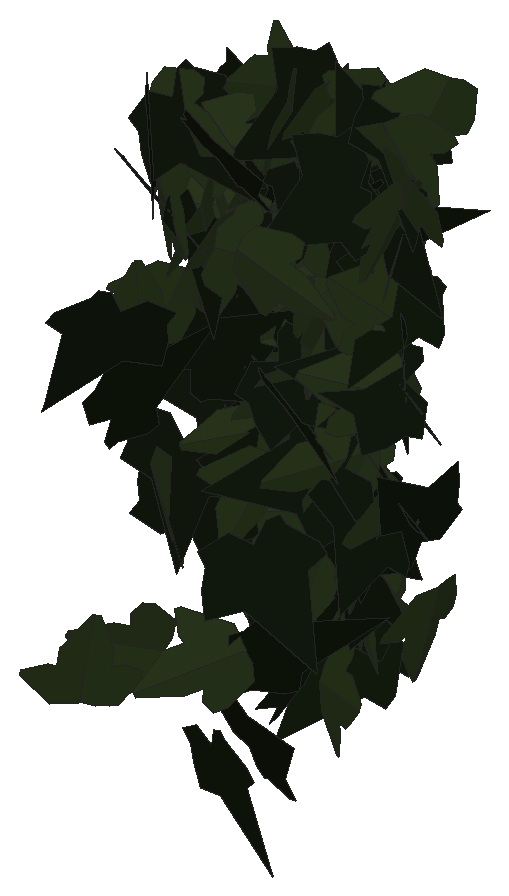
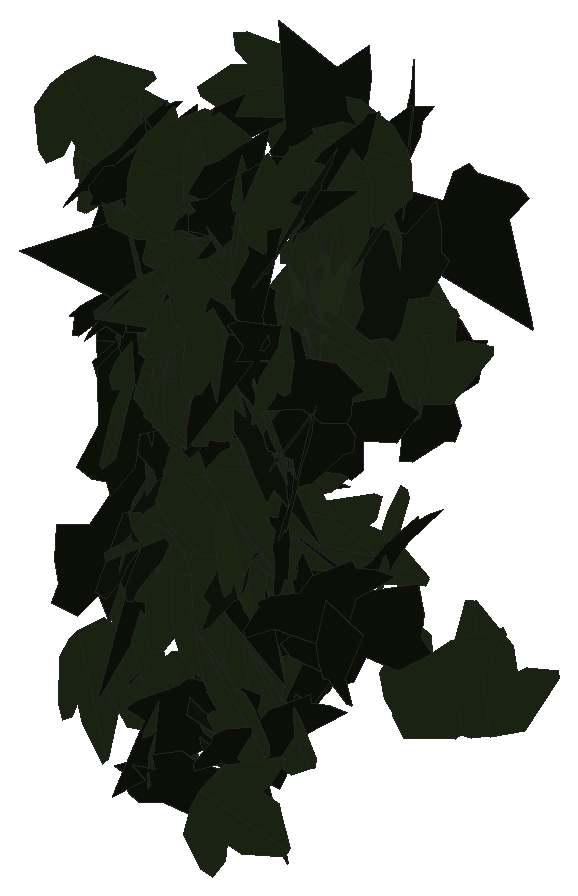
# SketchUp Ruby script. Lengths in inches.
U = 1.inch
M = Sketchup.active_model
def pt(a) = Geom::Point3d.new(a.map { |v| v * U })
def face(e, loops, mat)
  f = e.add_face(loops[0].map { |a| pt(a) })
  loops[1..].each { |l| e.add_face(l.map { |a| pt(a) }).erase! }
  f.material = f.back_material = mat if mat
  f
end
# faces: each face lists its corners as indices into pts; further lists are holes
def faces(e, pts, list, mat = nil) = list.each { |f| face(e, (f[0].is_a?(Array) ? f : [f]).map { |l| l.map { |i| pts[i] } }, mat) }
# xy, xz, yz: faces in a plane at the given z, y or x. An outline is a flat list of corners, or four numbers for a rectangle; further outlines are holes
def ring(l) = l.size == 4 ? [[l[0], l[1]], [l[2], l[1]], [l[2], l[3]], [l[0], l[3]]] : l.each_slice(2).to_a
def flat(e, list, mat, &to3) = list.each { |f| face(e, (f[0].is_a?(Array) ? f : [f]).map { |l| ring(l).map { |u, v| to3.(u, v) } }, mat) }
def xy(e, z, list, mat = nil) = flat(e, list, mat) { |x, y| [x, y, z] }
def xz(e, y, list, mat = nil) = flat(e, list, mat) { |x, z| [x, y, z] }
def yz(e, x, list, mat = nil) = flat(e, list, mat) { |y, z| [x, y, z] }
def lines(e, pts, list) = list.each { |a, b| e.add_line(pt(pts[a]), pt(pts[b])) }
# prism: a flat outline (further loops are holes) pulled along v
def prism(e, loops, v, mat = nil)
  f = face(e, loops, mat); d = Geom::Vector3d.new(v.map { |x| x * U })
  f.pushpull(f.normal.samedirection?(d) ? d.length : -d.length)
end
def box(e, o, s, mat = nil) = prism(e, [[o, [o[0] + s[0], o[1], o[2]], [o[0] + s[0], o[1] + s[1], o[2]], [o[0], o[1] + s[1], o[2]]]], [0, 0, s[2]], mat)
def at(x, y, z, deg = 0) = Geom::Transformation.translation(pt([x, y, z])) * Geom::Transformation.rotation(ORIGIN, Z_AXIS, deg.degrees)
def axes(o, x, y, z) = Geom::Transformation.new([*x, 0, *y, 0, *z, 0, *pt(o).to_a, 1])
def part(name) = M.definitions.add(name)
# library, detail: a bought-in or finely detailed component or shape, given as its bounding box
def library(name, o, s) = part(name).tap { |d| box(d.entities, o, s) }
def detail(e, o, s) = box(e.add_group.entities, o, s)
def put(e, d, t, mat = nil) = e.add_instance(d, t).tap { |i| i.material = mat if mat }
def group(e, t, mat = nil) = e.add_group.tap { |g| g.transformation = t; g.material = mat if mat }.entities
root = M.entities
M.materials.add("efeu1").color = [18, 25, 13]
M.materials.add("efeu2").color = [43, 57, 29]
c1 = part("ivyleaf_9")
p = [[1.54,2.16,1.25],[1.36,2.04,1.19],[-0.21,0.99,0.68],[-0.71,1.11,0.82],[-0.85,0.86,0.67],[-0.8,0.17,0.21],
  [-0.9,-0.01,0.1],[-0.67,-0.16,-0.02],[-0.08,-0.08,-0.05],[-0.03,-0.6,-0.4],[0.65,-0.88,-0.66],[0.83,-0.6,-0.49],
  [1.29,-0.42,-0.43],[1.8125,-0.07,-0.26],[1.21,0.44,0.15]]
faces(c1.entities,p,[[0,1,2,3,4,5,6,7,8,9,10,11,12,13,14]],"efeu1")
c2 = part("ivyleaf_10")
p = [[0,0.5,-0.03],[-0.0625,2.02,-0.43],[-0.19,2.01,-0.46],[-0.54,1.05,-0.29],[-0.52,0.625,-0.18],[-0.83,0.76,-0.28],
  [-1.16,0.64,-0.33],[-1.15,0.33,-0.24],[-0.77,-0.39,0.02],[-0.3,-0.51,0.16],[0.04,-0.48,0.23],[-0.02,2.01,-0.4375],
  [-0.06,2.01,-0.43],[0.04,-0.49,0.23],[0.67,-0.49,0.14],[1.38,0.36,-0.2],[1.375,0.51,-0.24],[0.81,0.65,-0.19],
  [0.62,0.59,-0.15],[0.6,1.09,-0.28],[0.5,1.23,-0.31]]
faces(c2.entities,p,[[0,1,2,3,4,5,6,7,8,9,10],[11,12,0,13,14,15,16,17,18,19,20]],"efeu2")
put(root,c1,axes([18.06,224.125,208.98],[-0.01391,0.03121,0.49883],[-0.2386,0.43807,-0.03406],[-0.43918,-0.23899,0.00271]))
put(root,c1,axes([17.82,224.65,209.74],[-0.1901,-0.4622,-0.01517],[0.00198,0.01558,-0.49975],[0.46245,-0.19007,-0.00409]))
put(root,c2,axes([17.95,222.78,211.19],[-0.31818,-0.37826,-0.07536],[-0.04879,-0.05744,0.49429],[-0.3826,0.3219,-0.00036]))
put(root,c2,axes([17.9,221.86,207.3],[-0.37151,-0.33269,0.03604],[0.02825,0.02248,0.49869],[-0.33344,0.37257,0.0021]))
put(root,c1,axes([17.58,223.4375,212.44],[0.12943,-0.28938,0.38666],[0.26736,-0.29043,-0.30686],[0.4022,0.28619,0.07956]))
put(root,c2,axes([17.55,224.12,212.06],[0.11112,-0.14043,-0.46683],[0.47707,-0.06718,0.13376],[-0.1003,-0.47515,0.11906]))
put(root,c2,axes([18.23,222.51,207.6],[-0.11023,-0.14853,-0.46453],[-0.2849,-0.36692,0.18493],[-0.39583,0.30546,-0.00374]))
put(root,c2,axes([18.21,223.04,211.77],[-0.26597,-0.38738,0.17088],[-0.08938,-0.14587,-0.46982],[0.41385,-0.28046,0.00835]))
put(root,c2,axes([18.04,224.69,212.23],[-0.00323,0.33062,-0.37508],[-0.01008,-0.37505,-0.33051],[-0.49989,0.00542,0.00909]))
put(root,c1,axes([17.93,223.48,209.53],[0.01314,-0.49109,0.09307],[0.01459,-0.09268,-0.49112],[0.49961,0.01562,0.0119]))
put(root,c1,axes([17.84,224.65,211.09],[0.13457,-0.07798,-0.4752],[0.43428,-0.19355,0.15474],[-0.20808,-0.45438,0.01564]))
put(root,c1,axes([17.99,223.54,208.6],[-0.22356,-0.06502,0.44248],[0.44577,-0.07247,0.21457],[0.03623,0.49043,0.09037]))
put(root,c1,axes([17.92,222.95,213.77],[0.05224,-0.08497,-0.48995],[0.46894,-0.15548,0.07696],[-0.16543,-0.46755,0.06345]))
put(root,c1,axes([17.8125,224.19,211.47],[0.40854,-0.13619,0.25406],[0.24568,-0.06599,-0.43045],[0.15077,0.47655,0.013]))
put(root,c2,axes([18.26,222.72,209.51],[-0.28195,0.40988,0.05002],[-0.02911,0.04069,-0.49749],[-0.41189,-0.28345,0.00092]))
put(root,c1,axes([17.95,224.48,212.09],[-0.05685,-0.19259,-0.4579],[0.34535,0.31598,-0.17577],[0.35708,-0.33626,0.0971]))
put(root,c1,axes([18.1,223.16,213.88],[0.15552,-0.30654,-0.3631],[-0.08133,0.35925,-0.33812],[0.46819,0.16423,0.06188]))
put(root,c2,axes([17.91,223.29,213.7],[-0.09678,0.01653,-0.49027],[0.45247,-0.19003,-0.09573],[-0.18949,-0.46219,0.02182]))
put(root,c1,axes([18.15,222.09,210.59],[0.04154,0.03134,0.49728],[0.33791,0.36495,-0.05123],[-0.36618,0.34033,0.00914]))
put(root,c1,axes([18.07,224.13,211.43],[0.29374,-0.39325,-0.09524],[-0.04492,0.08526,-0.49062],[0.40212,0.29679,0.01476]))
put(root,c2,axes([18.4,223.18,212.625],[0.0467,-0.41452,-0.27567],[-0.02682,0.27438,-0.41713],[0.49709,0.05374,0.0034]))
put(root,c2,axes([18.09,223.98,212.17],[-0.17648,-0.00632,0.46778],[0.38989,-0.27828,0.14333],[0.25854,0.41535,0.10315]))
put(root,c2,axes([18.08,223.06,212.8],[-0.11914,0.05053,-0.48296],[0.29143,-0.39033,-0.11273],[-0.38843,-0.30836,0.06355]))
put(root,c1,axes([18.47,224.61,211.29],[-0.37999,0.23331,-0.22622],[0.19248,-0.11886,-0.4459],[-0.26184,-0.42596,0.00052]))
put(root,c1,axes([18.14,224.44,213.35],[0.09216,-0.40164,0.28318],[0.04923,-0.27912,-0.4119],[0.48896,0.10381,-0.0119]))
put(root,c2,axes([18.4,223.83,212.2],[0.06041,-0.49434,0.04446],[0.0108,-0.04347,-0.49799],[0.49622,0.06113,0.00543]))
put(root,c1,axes([18.07,224.58,210.4375],[0.04402,-0.02574,-0.49739],[0.48753,-0.09992,0.04831],[-0.10189,-0.48924,0.0163]))
put(root,c2,axes([18.36,224.5625,213.52],[-0.05767,0.24345,0.4329],[0.11981,-0.41612,0.24997],[0.482,0.13256,-0.01034]))
put(root,c2,axes([18.39,224.48,211.45],[0.34023,-0.36262,0.05241],[0.03285,-0.04103,-0.49723],[0.36491,0.34179,-0.00409]))
put(root,c2,axes([18.53,224.34,211.49],[-0.37197,-0.32722,0.06757],[-0.04635,-0.04961,-0.49537],[0.33089,-0.37479,0.00658]))
put(root,c1,axes([18.62,221.54,212.18],[0.03438,0.26818,-0.42059],[-0.06367,-0.41578,-0.27032],[-0.49474,0.07215,0.00556]))
put(root,c2,axes([18.75,224.04,209.79],[-0.0862,-0.04576,0.49038],[-0.31876,-0.37432,-0.09096],[0.37545,-0.32831,0.03535]))
put(root,c2,axes([18.42,223.91,212.52],[0.22308,-0.36624,0.25711],[0.14635,-0.21177,-0.42864],[0.42287,0.2665,0.01271]))
put(root,c1,axes([18.3,223.34,212.4],[0.13837,-0.43133,0.21168],[0.0469,-0.20711,-0.45267],[0.47818,0.14513,-0.01686]))
put(root,c1,axes([18.46,224.53,208.05],[-0.15806,-0.47234,-0.04373],[0.0209,0.03912,-0.49803],[0.4739,-0.15926,0.00738]))
put(root,c1,axes([18.25,223.3,210.67],[-0.03073,-0.00895,0.49897],[0.49741,-0.04107,0.0299],[0.04045,0.49823,0.01143]))
put(root,c2,axes([18.65,224.83,207.3],[-0.12624,-0.30457,0.3759],[-0.01443,-0.38594,-0.31756],[0.48359,-0.09102,0.08865]))
put(root,c2,axes([18.3,223.48,213.35],[-0.08444,-0.07794,-0.48661],[0.43558,0.21914,-0.11069],[0.23053,-0.44261,0.03089]))
put(root,c2,axes([18.66,223.28,212.5],[0.12797,-0.48014,0.05555],[0.0076,-0.05546,-0.49686],[0.48329,0.12801,-0.0069]))
put(root,c2,axes([18.375,224.1,207.72],[0.37705,-0.15621,-0.28884],[0.26388,-0.11762,0.40808],[-0.19544,-0.46018,-0.00626]))
put(root,c2,axes([18.71,224.52,210.04],[0.10057,-0.48748,0.04741],[0.01077,-0.04618,-0.49775],[0.48966,0.10114,0.00121]))
put(root,c1,axes([18.94,224.45,213.06],[-0.18368,-0.12444,0.44808],[-0.38532,-0.22901,-0.22155],[0.26037,-0.4267,-0.01176]))
put(root,c1,axes([18.93,224.34,212.3],[0.14648,-0.14558,0.45536],[-0.24874,0.3835,0.20263],[-0.40825,-0.2859,0.03992]))
put(root,c2,axes([18.83,224.55,212.08],[-0.1472,-0.46998,0.08632],[-0.02027,-0.0841,-0.49246],[0.47741,-0.14848,0.0057]))
put(root,c2,axes([18.8,224.17,213.59],[0.08389,-0.38615,-0.30635],[-0.00954,0.30943,-0.39264],[0.49282,0.07172,0.04455]))
put(root,c2,axes([18.89,224.47,210.35],[0.44435,0.03637,-0.22634],[-0.22478,-0.02779,-0.44576],[-0.045,0.4979,-0.00834]))
put(root,c2,axes([18.52,224.59,208],[0.35812,-0.15987,-0.31015],[0.28195,-0.12922,0.39218],[-0.20555,-0.45579,-0.00241]))
put(root,c1,axes([18.65,224.49,212.13],[-0.28484,-0.17925,-0.36977],[0.31996,0.18558,-0.33643],[0.25786,-0.42829,0.00898]))
put(root,c1,axes([18.97,224.63,213.51],[-0.18501,-0.27509,0.3743],[-0.20926,-0.31034,-0.33151],[0.41471,-0.27931,-0.0003]))
put(root,c1,axes([18.86,224.32,212.35],[0.43281,0.14078,-0.20702],[-0.19613,-0.06631,-0.45512],[-0.1556,0.47517,-0.00218]))
put(root,c2,axes([19.02,224.51,212.73],[-0.24145,-0.33894,0.27717],[-0.06828,-0.28351,-0.40616],[0.43248,-0.23398,0.09062]))
put(root,c2,axes([18.82,223.14,212.35],[0.00931,-0.2776,-0.41575],[0.19873,0.38361,-0.25169],[0.45871,-0.16056,0.11748]))
put(root,c2,axes([19.12,224.55,210.09],[-0.23467,-0.22531,-0.37969],[-0.24908,-0.28747,0.32453],[-0.36454,0.34146,0.02268]))
put(root,c2,axes([19.02,224.82,211.61],[-0.02814,-0.15999,0.47288],[0.02645,-0.47344,-0.15861],[0.49851,0.01609,0.03511]))
put(root,c1,axes([18.72,224.34,209.63],[0.27871,-0.38288,0.1604],[0.09505,-0.1292,-0.47357],[0.40409,0.29447,0.00076]))
put(root,c1,axes([19.32,223.99,209.48],[0.13681,0.0602,-0.47714],[-0.44033,-0.18378,-0.14944],[-0.19337,0.46109,0.00273]))
put(root,c2,axes([18.82,223.87,208.45],[-0.04573,-0.01926,-0.49753],[0.32055,-0.38345,-0.01462],[-0.38099,-0.32031,0.04742]))
put(root,c2,axes([19.23,223.25,209.76],[-0.22513,-0.38611,0.22413],[-0.06689,-0.21901,-0.44448],[0.44141,-0.23012,0.04696]))
put(root,c2,axes([19.17,224.38,213.8],[0.05287,-0.4972,0.00042],[-0.00039,-0.00046,-0.5],[0.4972,0.05287,-0.00044]))
put(root,c2,axes([19.48,224.52,211.39],[0.11406,0.09201,-0.47804],[-0.47672,-0.07834,-0.12883],[-0.0986,0.48518,0.06985]))
put(root,c1,axes([18.85,223,213.49],[0.00147,-0.2279,0.44504],[0.31332,-0.3464,-0.17842],[0.38965,0.27941,0.14179]))
put(root,c2,axes([19,224.33,212.47],[-0.29899,-0.20363,-0.34517],[0.30185,0.16885,-0.36108],[0.26362,-0.42429,0.02196]))
put(root,c2,axes([19.25,223.91,209.9],[0.16636,-0.46218,-0.09333],[-0.0312,0.08796,-0.49121],[0.47048,0.16926,0.00042]))
put(root,c2,axes([19.22,224.29,211.43],[-0.13452,-0.29638,0.37956],[0.1126,-0.40252,-0.2744],[0.46821,0.01165,0.17504]))
put(root,c1,axes([19.53,223.65,207.39],[-0.28898,0.40736,0.02331],[-0.01352,0.01899,-0.49946],[-0.40781,-0.2893,0.00004]))
put(root,c2,axes([19.18,224.56,211.28],[-0.096,0.38894,-0.29918],[0.05583,-0.29421,-0.4004],[-0.48751,-0.11028,0.01306]))
put(root,c2,axes([19.37,224.46,209.17],[-0.12926,-0.46906,0.11522],[-0.03419,-0.11009,-0.48653],[0.48179,-0.13365,-0.00362]))
put(root,c2,axes([19.5,224.41,211.27],[0.06599,0.07364,-0.49013],[-0.35404,-0.33902,-0.0986],[-0.34685,0.36006,0.0074]))
put(root,c1,axes([19.46,223.68,207.57],[-0.34191,0.28777,-0.22424],[-0.16989,0.14638,0.44689],[0.32285,0.38179,-0.00232]))
put(root,c2,axes([19.25,223.85,207.76],[-0.3407,-0.35144,0.10205],[0.06938,0.07487,0.48947],[-0.35932,0.34768,-0.00224]))
put(root,c1,axes([19.12,224.41,208.04],[0.03068,-0.2969,-0.40114],[0.09241,0.39832,-0.28775],[0.49043,-0.05648,0.07931]))
put(root,c2,axes([19.46,224.74,213.67],[-0.04066,-0.24872,0.43184],[-0.06656,-0.42668,-0.25201],[0.49388,-0.07798,0.00158]))
put(root,c1,axes([19.52,224.61,207.25],[-0.45889,-0.19611,0.03101],[-0.02762,-0.01428,-0.49903],[0.19661,-0.45971,0.00228]))
put(root,c2,axes([19.49,223.35,210.92],[-0.14609,-0.4746,-0.05844],[0.01894,0.05532,-0.49657],[0.47781,-0.1473,0.00182]))
put(root,c2,axes([19.11,223.63,209.11],[0.09403,-0.00935,-0.49099],[0.49026,-0.02713,0.0944],[-0.02841,-0.49918,0.00406]))
put(root,c2,axes([19.46,223.99,209.81],[0.05752,0.42974,0.24903],[0.00623,0.25005,-0.43294],[-0.49664,0.0529,0.02341]))
put(root,c2,axes([19.83,221.8,208.36],[-0.17647,-0.08274,0.46045],[-0.2877,-0.36886,-0.17655],[0.3689,-0.32725,0.08258]))
put(root,c2,axes([19.27,224.31,211.47],[0.35642,-0.03769,0.34863],[0.34816,-0.0212,-0.35824],[0.04179,0.49813,0.01113]))
put(root,c2,axes([19.5,223.92,211.44],[0.20464,-0.39763,0.22363],[0.12989,-0.18417,-0.44633],[0.43732,0.24077,0.02792]))
put(root,c2,axes([19.52,223.76,211.7],[-0.02955,0.44421,-0.2276],[0.01879,-0.22685,-0.44518],[-0.49877,-0.03487,-0.00329]))
put(root,c2,axes([19.61,224.33,207.99],[-0.21593,0.44443,0.07651],[-0.04346,0.06393,-0.49399],[-0.44887,-0.21998,0.01102]))
put(root,c1,axes([19.58,223.93,212.8],[-0.34404,0.30144,0.20193],[0.15339,-0.13134,0.45741],[0.3288,0.37668,-0.0021]))
put(root,c2,axes([19.5,224.23,212.9],[0.36567,0.32207,0.11207],[0.07977,0.07898,-0.48724],[-0.33155,0.37421,0.00638]))
put(root,c1,axes([19.46,223.27,211.13],[0.17521,-0.2168,-0.41509],[-0.02659,0.43787,-0.23992],[0.46754,0.10614,0.14191]))
put(root,c2,axes([19.44,224.14,212.28],[-0.08703,-0.09898,-0.48232],[0.35538,0.32637,-0.1311],[0.34078,-0.36563,0.01354]))
put(root,c1,axes([19.96,223.59,209.9],[-0.08083,-0.1992,-0.45143],[-0.19853,-0.40565,0.21455],[-0.45172,0.21393,-0.01351]))
put(root,c1,axes([19.46,224.44,210.7],[-0.08295,-0.16367,0.46512],[0.21337,-0.43712,-0.11576],[0.44451,0.17928,0.14236]))
put(root,c2,axes([19.83,223.92,211.48],[-0.13951,0.45102,-0.16467],[-0.05894,0.15409,0.472],[0.47651,0.15111,0.01017]))
put(root,c2,axes([19.68,223.89,209.16],[-0.3346,-0.32874,0.17314],[0.12556,0.11925,0.46906],[-0.34969,0.35737,0.00275]))
put(root,c2,axes([19.46,224.57,209.36],[-0.15448,0.06763,-0.4707],[0.42094,-0.21081,-0.16844],[-0.22124,-0.44831,0.0082]))
put(root,c2,axes([19.55,223.99,206.96],[0.04014,-0.12573,-0.48227],[0.32658,-0.35884,0.12074],[-0.37647,-0.32469,0.05331]))
put(root,c1,axes([19.52,223.27,210.7],[0.1759,-0.33052,0.33138],[0.21469,-0.25759,-0.37088],[0.41589,0.27277,0.0513]))
put(root,c2,axes([19.93,223.625,210],[0.00336,0.04745,0.49773],[-0.01291,-0.49757,0.04753],[0.49982,-0.01318,-0.00212]))
put(root,c1,axes([20.09,224.25,213.02],[-0.36083,-0.32881,0.10807],[0.08658,0.06541,0.48808],[-0.33511,0.37095,0.00974]))
put(root,c2,axes([19.74,224.51,207.92],[-0.4226,-0.01688,0.26668],[0.26721,-0.02945,0.42158],[0.00147,0.49885,0.03391]))
put(root,c1,axes([19.65,221.88,207.14],[0.30718,-0.39407,0.01871],[0.01178,-0.01455,-0.49965],[0.39433,0.30741,0.00035]))
put(root,c1,axes([20.03,223.77,213.24],[-0.23591,-0.27691,0.34303],[-0.168,-0.30323,-0.36032],[0.40759,-0.28526,0.05003]))
put(root,c1,axes([19.95,224.58,209.21],[0.31798,-0.37904,0.07222],[-0.03007,0.06896,0.49431],[-0.38468,-0.31871,0.02107]))
put(root,c1,axes([19.79,224.3,208.34],[-0.03146,-0.37819,0.32555],[0.08068,-0.32576,-0.37064],[0.49244,0.02921,0.08152]))
put(root,c1,axes([20,224.05,209.15],[0.15054,-0.15674,-0.4503],[-0.31639,0.32043,-0.2173],[0.3567,0.35037,-0.0027]))
put(root,c1,axes([19.68,224.17,212.36],[0.21016,0.06627,0.44882],[0.42271,0.15103,-0.22023],[-0.16476,0.47201,0.00745]))
put(root,c1,axes([19.85,224.43,212.21],[0.06748,-0.49482,-0.02448],[0.00047,0.02477,-0.49939],[0.49543,0.06737,0.00381]))
put(root,c1,axes([19.79,222.33,207.05],[-0.02002,-0.12847,0.4828],[0.30063,-0.38901,-0.09104],[0.39902,0.28664,0.09282]))
put(root,c2,axes([20.12,224.29,208.96],[0.03509,0.11146,-0.48615],[-0.08959,-0.47802,-0.11606],[-0.49066,0.09525,-0.01357]))
put(root,c2,axes([20.23,224.21,212.54],[0.27749,-0.37907,-0.17118],[-0.0889,0.14697,-0.46957],[0.40632,0.29104,0.01416]))
put(root,c1,axes([19.97,224.65,213.68],[0.06912,-0.49407,0.03339],[0.00576,-0.03291,-0.49888],[0.49517,0.06935,0.00114]))
put(root,c1,axes([19.91,224.125,212.88],[-0.11842,-0.12845,-0.46848],[0.34721,0.31486,-0.17409],[0.33974,-0.36655,0.01462]))
put(root,c2,axes([20.21,223.95,210.96],[-0.05292,-0.32136,-0.37937],[0.04797,0.37644,-0.32557],[0.49487,-0.07086,-0.00901]))
put(root,c1,axes([20.0625,222.0625,209.625],[-0.01063,-0.3671,-0.3393],[0.06249,0.33574,-0.3652],[0.49597,-0.05017,0.03874]))
put(root,c1,axes([19.99,222.2,208.2],[0.16951,0.10164,0.45928],[0.39562,0.23329,-0.19764],[-0.25447,0.4304,-0.00133]))
put(root,c2,axes([20.22,224.1875,213.74],[-0.41659,-0.21555,-0.17319],[0.15027,0.0864,-0.46899],[0.23211,-0.4428,-0.00721]))
put(root,c1,axes([19.92,224.46,210.64],[0.37878,-0.05886,-0.32103],[0.31423,-0.06717,0.38308],[-0.08822,-0.49196,-0.0139]))
put(root,c2,axes([20.3,223.86,211.79],[-0.08169,0.35714,0.34026],[0.05437,-0.33628,0.36601],[0.49028,0.09679,0.0161]))
put(root,c1,axes([20.04,224.3,211.38],[-0.11719,-0.01761,-0.48575],[0.48569,-0.02396,-0.11631],[-0.01919,-0.49911,0.02272]))
put(root,c1,axes([20.29,224.37,211.96],[-0.15712,-0.43097,0.19894],[-0.06986,-0.18627,-0.45872],[0.4695,-0.17194,-0.00168]))
put(root,c2,axes([20.3,223.84,209.29],[0.12315,-0.42875,0.22584],[0.0921,-0.20807,-0.44523],[0.47576,0.15126,0.02773]))
put(root,c2,axes([20.43,224.69,214.09],[-0.22568,-0.37882,0.23572],[-0.04174,-0.24507,-0.43382],[0.44421,-0.21549,0.07899]))
put(root,c1,axes([20.19,223.83,209.36],[-0.05949,-0.43349,0.24197],[0.0285,-0.24628,-0.43421],[0.49563,-0.03787,0.05401]))
put(root,c2,axes([20.46,223.58,211.01],[0.02551,0.25296,0.43053],[-0.07889,-0.42364,0.25359],[0.49308,-0.08087,0.01829]))
put(root,c1,axes([20.36,224.45,208.83],[0.13949,0.17605,0.44671],[-0.27218,-0.35423,0.2246],[0.39555,-0.30582,-0.00299]))
put(root,c2,axes([20.41,224.05,213.09],[0.05457,-0.45019,0.2106],[0.01109,-0.21071,-0.4533],[0.49689,0.05415,-0.01301]))
put(root,c2,axes([20.67,223.93,213.35],[-0.39578,0.0869,0.29292],[-0.28485,0.06846,-0.40519],[-0.11053,-0.48761,-0.00469]))
put(root,c2,axes([20.48,224.49,208.07],[-0.00139,-0.49959,0.02014],[-0.0002,-0.02014,-0.49959],[0.5,-0.00139,-0.00014]))
put(root,c1,axes([20.61,223.8125,211.08],[-0.03997,-0.4084,-0.28568],[-0.03441,-0.28365,0.41031],[-0.49721,0.05246,-0.00543]))
put(root,c2,axes([20.12,222.05,213.14],[-0.20108,0.04718,-0.45535],[0.44733,-0.08544,-0.20639],[-0.09728,-0.49038,-0.00785]))
